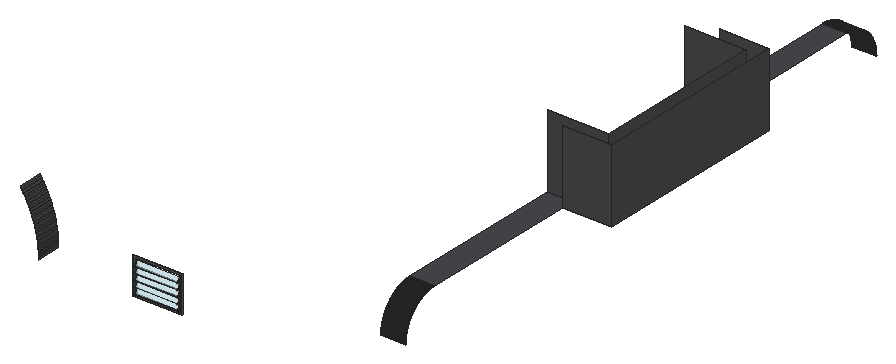
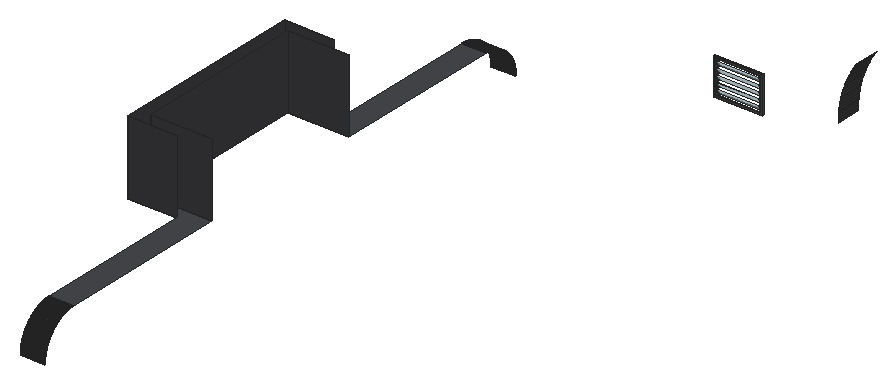
# SketchUp Ruby script. Lengths in inches.
U = 1.inch
M = Sketchup.active_model
def pt(a) = Geom::Point3d.new(a.map { |v| v * U })
def face(e, loops, mat)
  f = e.add_face(loops[0].map { |a| pt(a) })
  loops[1..].each { |l| e.add_face(l.map { |a| pt(a) }).erase! }
  f.material = f.back_material = mat if mat
  f
end
# faces: each face lists its corners as indices into pts; further lists are holes
def faces(e, pts, list, mat = nil) = list.each { |f| face(e, (f[0].is_a?(Array) ? f : [f]).map { |l| l.map { |i| pts[i] } }, mat) }
# xy, xz, yz: faces in a plane at the given z, y or x. An outline is a flat list of corners, or four numbers for a rectangle; further outlines are holes
def ring(l) = l.size == 4 ? [[l[0], l[1]], [l[2], l[1]], [l[2], l[3]], [l[0], l[3]]] : l.each_slice(2).to_a
def flat(e, list, mat, &to3) = list.each { |f| face(e, (f[0].is_a?(Array) ? f : [f]).map { |l| ring(l).map { |u, v| to3.(u, v) } }, mat) }
def xy(e, z, list, mat = nil) = flat(e, list, mat) { |x, y| [x, y, z] }
def xz(e, y, list, mat = nil) = flat(e, list, mat) { |x, z| [x, y, z] }
def yz(e, x, list, mat = nil) = flat(e, list, mat) { |y, z| [x, y, z] }
def lines(e, pts, list) = list.each { |a, b| e.add_line(pt(pts[a]), pt(pts[b])) }
# prism: a flat outline (further loops are holes) pulled along v
def prism(e, loops, v, mat = nil)
  f = face(e, loops, mat); d = Geom::Vector3d.new(v.map { |x| x * U })
  f.pushpull(f.normal.samedirection?(d) ? d.length : -d.length)
end
def box(e, o, s, mat = nil) = prism(e, [[o, [o[0] + s[0], o[1], o[2]], [o[0] + s[0], o[1] + s[1], o[2]], [o[0], o[1] + s[1], o[2]]]], [0, 0, s[2]], mat)
def at(x, y, z, deg = 0) = Geom::Transformation.translation(pt([x, y, z])) * Geom::Transformation.rotation(ORIGIN, Z_AXIS, deg.degrees)
def axes(o, x, y, z) = Geom::Transformation.new([*x, 0, *y, 0, *z, 0, *pt(o).to_a, 1])
def part(name) = M.definitions.add(name)
# library, detail: a bought-in or finely detailed component or shape, given as its bounding box
def library(name, o, s) = part(name).tap { |d| box(d.entities, o, s) }
def detail(e, o, s) = box(e.add_group.entities, o, s)
def put(e, d, t, mat = nil) = e.add_instance(d, t).tap { |i| i.material = mat if mat }
def group(e, t, mat = nil) = e.add_group.tap { |g| g.transformation = t; g.material = mat if mat }.entities
root = M.entities
M.materials.add("1432 AP 8245 TAR ROAD").color = [71, 72, 75]
M.materials.add("[Color M05]").color = [114, 114, 114]
M.materials.add("[Color M06]").color = [86, 86, 86]
M.materials.add("[Color M09]").color = [0, 0, 0]
M.materials.add("[Translucent Glass Safety]").color = [204, 235, 244]
M.materials["[Translucent Glass Safety]"].alpha = 0.5
M.materials.add("[Translucent Resin Crush Gray]").color = [209, 209, 209]
M.materials["[Translucent Resin Crush Gray]"].alpha = 0.8
c1 = part("Louvre blade clip")
prism(c1.entities,[[[0,0.85,29.12],[0,5.29,29.12],[0,5.29,0],[0,0,0],[0,0,9.17],[0,0.85,9.17],[0,0.85,0.85],[0,4.45,0.85],[0,4.45,28.27],[0,0.85,28.27]]],[0.5625,0,0],"[Color M09]")
c2 = part("Glass louvre blade")
p = [[0.14,0.43,0.55],[0.14,2.01,6.46],[0,2.375,6.37],[0,0.79,0.45],[29.62,0.79,0.45],[29.77,0.43,0.55],
  [29.77,2.01,6.46],[29.62,2.375,6.37]]
faces(c2.entities,p,[[0,1,2,3],[1,0,5,6],[4,7,6,5],[3,2,7,4],[2,1,6,7]],"[Translucent Glass Safety]")
faces(c2.entities,p,[[3,4,5,0]],"[Translucent Resin Crush Gray]")
put(c2.entities,c1,axes([29.2,0,0.28],[1,0,0],[0,0.19968,-0.0535],[0,0.06043,0.22552]))
put(c2.entities,c1,axes([-0.09,0.05,0.6],[1,0,0],[0,0.19968,-0.0535],[0,0.06043,0.22552]))
c3 = part("Window frame")
prism(c3.entities,[[[28.75,1.1875,0],[0,1.1875,0],[0,1.1875,36],[28.75,1.1875,36]],[[27.3,1.1875,1.45],[27.3,1.1875,34.55],[1.45,1.1875,34.55],[1.45,1.1875,1.45]]],[0,-1.1875,0],"[Color M06]")
c4 = part("Louvred window")
put(c4.entities,c2,axes([1.64,0,14.6],[0.837,0,0],[0,1,0],[0,0,0.7998]))
put(c4.entities,c2,axes([1.64,0,8.29],[0.837,0,0],[0,1,0],[0,0,0.7998]))
put(c4.entities,c2,axes([1.64,0,20.72],[0.837,0,0],[0,1,0],[0,0,0.7998]))
put(c4.entities,c2,axes([1.64,0,26.97],[0.837,0,0],[0,1,0],[0,0,0.7998]))
put(c4.entities,c2,axes([1.64,0,2.47],[0.837,0,0],[0,1,0],[0,0,0.7998]))
put(c4.entities,c3,axes([0,1.37,0],[0.98,0,0],[0,1,0],[0,0,1]),"[Color M05]")
c5 = part("BathRoom Window")
put(c5.entities,c4,at(2.44,2.32,-1.4375))
xy(root,419.79,[[573,160.9,585,161.13],[573,161.13,585,161.37],[573,161.37,573,245.37,603,245.37,603,329.37,573,329.37,573,413.37,585,413.37,585,335.37,609,335.37,609,239.37,585,239.37,585,161.37],[573,413.37,585,413.61],[573,413.61,585,413.84]],"1432 AP 8245 TAR ROAD")
xz(root,143.37,[[573,401.79,585,402.03]],"1432 AP 8245 TAR ROAD")
xz(root,239.37,[[585,419.79,609,455.79]],"1432 AP 8245 TAR ROAD")
xz(root,245.37,[[573,419.79,603,455.79]],"1432 AP 8245 TAR ROAD")
xz(root,329.37,[[573,419.79,603,455.79]],"1432 AP 8245 TAR ROAD")
xz(root,335.37,[[585,419.79,609,455.79]],"1432 AP 8245 TAR ROAD")
xz(root,431.36,[[573,402.26,585,402.5]],"1432 AP 8245 TAR ROAD")
xz(root,431.37,[[573,401.79,585,402.03]],"1432 AP 8245 TAR ROAD")
yz(root,444,[[95.37,410.79,107.37,411.46]],"1432 AP 8245 TAR ROAD")
yz(root,603,[[245.37,419.79,329.37,455.79]],"1432 AP 8245 TAR ROAD")
yz(root,609,[[239.37,419.79,335.37,455.79]],"1432 AP 8245 TAR ROAD")
p = [[573,143.37,402.03],[573,143.375,402.26],[585,143.375,402.26],[585,143.37,402.03],[573,431.36,402.26],[573,431.37,402.03],
  [585,431.37,402.03],[585,431.36,402.26],[573,143.38,402.5],[585,143.38,402.5],[573,143.39,402.73],[585,143.39,402.73],
  [573,431.35,402.73],[573,431.36,402.5],[585,431.36,402.5],[585,431.35,402.73],[573,143.41,402.97],[585,143.41,402.97],
  [573,431.33,402.97],[585,431.33,402.97],[573,143.43,403.2],[585,143.43,403.2],[573,431.3125,403.2],[585,431.3125,403.2],
  [573,143.45,403.4375],[585,143.45,403.4375],[573,431.29,403.4375],[585,431.29,403.4375],[573,143.47,403.67],[585,143.47,403.67],
  [573,431.27,403.67],[585,431.27,403.67],[573,143.49,403.91],[585,143.49,403.91],[573,431.25,403.91],[585,431.25,403.91],
  [573,143.52,404.14],[585,143.52,404.14],[573,431.22,404.14],[585,431.22,404.14],[573,143.56,404.375],[585,143.56,404.375],
  [573,431.18,404.375],[585,431.18,404.375],[573,143.59,404.61],[585,143.59,404.61],[573,431.15,404.61],[585,431.15,404.61],
  [573,143.63,404.84],[585,143.63,404.84],[573,431.11,404.84],[585,431.11,404.84],[573,143.67,405.07],[585,143.67,405.07],
  [573,431.07,405.07],[585,431.07,405.07],[573,143.72,405.3],[585,143.72,405.3],[573,431.02,405.3],[585,431.02,405.3],
  [573,143.76,405.53],[585,143.76,405.53],[573,430.98,405.53],[585,430.98,405.53],[573,143.8125,405.76],[585,143.8125,405.76],
  [573,430.93,405.76],[585,430.93,405.76],[573,143.87,405.99],[585,143.87,405.99],[573,430.87,405.99],[585,430.87,405.99],
  [573,143.92,406.22],[585,143.92,406.22],[573,430.82,406.22],[585,430.82,406.22],[573,143.98,406.45],[585,143.98,406.45],
  [573,430.76,406.45],[585,430.76,406.45],[573,144.05,406.68],[585,144.05,406.68],[573,430.69,406.68],[585,430.69,406.68],
  [573,144.11,406.9],[585,144.11,406.9],[573,430.63,406.9],[585,430.63,406.9],[573,144.18,407.13],[585,144.18,407.13],
  [573,430.56,407.13],[585,430.56,407.13],[573,144.25,407.35],[585,144.25,407.35],[573,430.49,407.35],[585,430.49,407.35],
  [573,144.33,407.58],[585,144.33,407.58],[573,430.41,407.58],[585,430.41,407.58],[573,144.4,407.8],[585,144.4,407.8],
  [573,430.34,407.8],[585,430.34,407.8],[573,144.48,408.02],[585,144.48,408.02],[573,430.26,408.02],[585,430.26,408.02],
  [573,144.57,408.24],[585,144.57,408.24],[573,430.17,408.24],[585,430.17,408.24],[573,144.65,408.46],[585,144.65,408.46],
  [573,430.09,408.46],[585,430.09,408.46],[573,144.74,408.68],[585,144.74,408.68],[573,430,408.68],[585,430,408.68],
  [573,144.83,408.9],[585,144.83,408.9],[573,429.91,408.9],[585,429.91,408.9],[573,144.93,409.11],[585,144.93,409.11],
  [573,429.8125,409.11],[585,429.8125,409.11],[573,145.02,409.33],[585,145.02,409.33],[573,429.72,409.33],[585,429.72,409.33],
  [573,145.125,409.54],[585,145.125,409.54],[573,429.62,409.54],[585,429.62,409.54],[573,145.23,409.75],[585,145.23,409.75],
  [573,429.51,409.75],[585,429.51,409.75],[573,145.33,409.96],[585,145.33,409.96],[573,429.41,409.96],[585,429.41,409.96],
  [573,145.44,410.17],[585,145.44,410.17],[573,429.3,410.17],[585,429.3,410.17],[573,145.55,410.38],[585,145.55,410.38],
  [573,429.1875,410.38],[585,429.1875,410.38],[573,145.67,410.59],[585,145.67,410.59],[573,429.07,410.59],[585,429.07,410.59],
  [573,145.78,410.79],[585,145.78,410.79],[573,428.96,410.79],[585,428.96,410.79],[573,145.9,411],[585,145.9,411],
  [573,428.84,411],[585,428.84,411],[573,146.02,411.2],[585,146.02,411.2],[573,428.72,411.2],[585,428.72,411.2],
  [573,146.15,411.4],[585,146.15,411.4],[573,428.59,411.4],[585,428.59,411.4],[573,146.27,411.6],[585,146.27,411.6],
  [573,428.47,411.6],[585,428.47,411.6],[444,107.37,411.46],[443.98,107.37,412.13],[443.98,95.37,412.13],[444,95.37,411.46],
  [573,146.4,411.79],[585,146.4,411.79],[573,428.34,411.79],[585,428.34,411.79],[573,146.54,411.99],[585,146.54,411.99],
  [573,428.2,411.99],[585,428.2,411.99],[573,146.67,412.18],[585,146.67,412.18],[573,428.07,412.18],[585,428.07,412.18],
  [443.96,107.37,412.79],[443.96,95.37,412.79],[573,146.81,412.37],[585,146.81,412.37],[573,427.93,412.37],[585,427.93,412.37],
  [573,146.95,412.5625],[585,146.95,412.5625],[573,427.79,412.5625],[585,427.79,412.5625],[573,147.09,412.75],[585,147.09,412.75],
  [573,427.65,412.75],[585,427.65,412.75],[573,147.23,412.9375],[585,147.23,412.9375],[573,427.51,412.9375],[585,427.51,412.9375],
  [443.93,107.37,413.46],[443.93,95.37,413.46],[573,147.38,413.12],[585,147.38,413.12],[573,427.36,413.12],[585,427.36,413.12],
  [573,147.53,413.3],[585,147.53,413.3],[573,427.21,413.3],[585,427.21,413.3],[573,147.68,413.48],[585,147.68,413.48],
  [573,427.06,413.48],[585,427.06,413.48],[443.89,107.37,414.13],[443.89,95.37,414.13],[573,147.84,413.66],[585,147.84,413.66],
  [573,426.9,413.66],[585,426.9,413.66],[573,147.99,413.84],[585,147.99,413.84],[573,426.75,413.84],[585,426.75,413.84],
  [573,148.15,414.01],[585,148.15,414.01],[573,426.59,414.01],[585,426.59,414.01],[573,148.3125,414.18],[585,148.3125,414.18],
  [573,426.43,414.18],[585,426.43,414.18],[443.84,107.37,414.79],[443.84,95.37,414.79],[573,148.48,414.35],[585,148.48,414.35],
  [573,426.26,414.35],[585,426.26,414.35],[573,148.64,414.52],[585,148.64,414.52],[573,426.1,414.52],[585,426.1,414.52],
  [573,148.81,414.69],[585,148.81,414.69],[573,425.93,414.69],[585,425.93,414.69],[573,148.98,414.85],[585,148.98,414.85],
  [573,425.76,414.85],[585,425.76,414.85],[443.79,107.37,415.46],[443.79,95.37,415.46],[573,149.15,415.01],[585,149.15,415.01],
  [573,425.59,415.01],[585,425.59,415.01],[573,149.33,415.17],[585,149.33,415.17],[573,425.41,415.17],[585,425.41,415.17],
  [573,149.5,415.33],[585,149.5,415.33],[573,425.24,415.33],[585,425.24,415.33],[573,149.68,415.48],[585,149.68,415.48],
  [573,425.06,415.48],[585,425.06,415.48],[443.72,107.37,416.125],[443.72,95.37,416.125],[573,149.86,415.63],[585,149.86,415.63],
  [573,424.88,415.63],[585,424.88,415.63],[573,150.04,415.78],[585,150.04,415.78],[573,424.7,415.78],[585,424.7,415.78],
  [573,150.23,415.93],[585,150.23,415.93],[573,424.51,415.93],[585,424.51,415.93],[573,150.41,416.07],[585,150.41,416.07],
  [573,424.33,416.07],[585,424.33,416.07],[443.65,107.37,416.79],[443.65,95.37,416.79],[573,150.6,416.21],[585,150.6,416.21],
  [573,424.14,416.21],[585,424.14,416.21],[573,150.79,416.35],[585,150.79,416.35],[573,423.95,416.35],[585,423.95,416.35],
  [573,150.98,416.49],[585,150.98,416.49],[573,423.76,416.49],[585,423.76,416.49],[573,151.17,416.625],[585,151.17,416.625],
  [573,423.57,416.625],[585,423.57,416.625],[573,151.37,416.76],[585,151.37,416.76],[573,423.37,416.76],[585,423.37,416.76],
  [443.5625,107.37,417.45],[443.5625,95.37,417.45],[573,151.57,416.89],[585,151.57,416.89],[573,423.17,416.89],[585,423.17,416.89],
  [573,151.76,417.02],[585,151.76,417.02],[573,422.97,417.02],[585,422.97,417.02],[573,151.96,417.14],[585,151.96,417.14],
  [573,422.77,417.14],[585,422.77,417.14],[573,152.17,417.26],[585,152.17,417.26],[573,422.57,417.26],[585,422.57,417.26],
  [573,152.37,417.38],[585,152.37,417.38],[573,422.37,417.38],[585,422.37,417.38],[443.47,107.37,418.11],[443.47,95.37,418.11],
  [573,152.57,417.5],[585,152.57,417.5],[573,422.17,417.5],[585,422.17,417.5],[573,152.78,417.61],[585,152.78,417.61],
  [573,421.96,417.61],[585,421.96,417.61],[573,152.99,417.72],[585,152.99,417.72],[573,421.75,417.72],[585,421.75,417.72],
  [573,153.2,417.83],[585,153.2,417.83],[573,421.54,417.83],[585,421.54,417.83],[573,153.41,417.9375],[585,153.41,417.9375],
  [573,421.33,417.9375],[585,421.33,417.9375],[573,153.62,418.04],[585,153.62,418.04],[573,421.12,418.04],[585,421.12,418.04],
  [573,153.83,418.14],[585,153.83,418.14],[573,420.91,418.14],[585,420.91,418.14],[443.37,107.37,418.77],[443.37,95.37,418.77],
  [573,154.05,418.24],[585,154.05,418.24],[573,420.69,418.24],[585,420.69,418.24],[573,154.26,418.33],[585,154.26,418.33],
  [573,420.48,418.33],[585,420.48,418.33],[573,154.48,418.42],[585,154.48,418.42],[573,420.26,418.42],[585,420.26,418.42],
  [573,154.7,418.51],[585,154.7,418.51],[573,420.04,418.51],[585,420.04,418.51],[573,154.92,418.6],[585,154.92,418.6],
  [573,419.82,418.6],[585,419.82,418.6],[573,155.14,418.68],[585,155.14,418.68],[573,419.6,418.68],[585,419.6,418.68],
  [573,155.36,418.76],[585,155.36,418.76],[573,419.38,418.76],[585,419.38,418.76],[443.26,107.37,419.43],[443.26,95.37,419.43],
  [573,155.58,418.84],[585,155.58,418.84],[573,155.81,418.91],[585,155.81,418.91],[573,418.93,418.91],[573,419.16,418.84],
  [585,419.16,418.84],[585,418.93,418.91],[573,156.03,418.98],[585,156.03,418.98],[573,418.71,418.98],[585,418.71,418.98],
  [573,156.26,419.05],[585,156.26,419.05],[573,418.48,419.05],[585,418.48,419.05],[573,156.48,419.12],[585,156.48,419.12],
  [573,156.71,419.18],[585,156.71,419.18],[573,418.03,419.18],[573,418.26,419.12],[585,418.26,419.12],[585,418.03,419.18],
  [573,156.9375,419.24],[585,156.9375,419.24],[573,157.17,419.29],[585,157.17,419.29],[573,417.57,419.29],[573,417.8,419.24],
  [585,417.8,419.24],[585,417.57,419.29],[573,157.4,419.35],[585,157.4,419.35],[573,157.63,419.4],[585,157.63,419.4],
  [573,417.11,419.4],[573,417.34,419.35],[585,417.34,419.35],[585,417.11,419.4],[443.15,107.37,420.09],[443.15,95.37,420.09],
  [573,157.86,419.45],[585,157.86,419.45],[573,158.09,419.49],[585,158.09,419.49],[573,416.65,419.49],[573,416.88,419.45],
  [585,416.88,419.45],[585,416.65,419.49],[573,158.32,419.53],[585,158.32,419.53],[573,158.55,419.57],[585,158.55,419.57],
  [573,416.1875,419.57],[573,416.42,419.53],[585,416.42,419.53],[585,416.1875,419.57],[573,158.79,419.61],[585,158.79,419.61],
  [573,159.02,419.64],[585,159.02,419.64],[573,159.25,419.67],[585,159.25,419.67],[573,415.49,419.67],[573,415.72,419.64],
  [585,415.72,419.64],[585,415.49,419.67],[573,415.95,419.61],[585,415.95,419.61],[573,159.49,419.69],[585,159.49,419.69],
  [573,159.72,419.72],[585,159.72,419.72],[573,159.96,419.74],[585,159.96,419.74],[573,160.19,419.75],[585,160.19,419.75],
  [573,414.55,419.75],[573,414.78,419.74],[585,414.78,419.74],[585,414.55,419.75],[573,415.02,419.72],[585,415.02,419.72],
  [573,415.25,419.69],[585,415.25,419.69],[573,160.43,419.77],[585,160.43,419.77],[573,160.66,419.78],[585,160.66,419.78],
  [573,160.9,419.79],[585,160.9,419.79],[573,413.84,419.79],[573,414.08,419.78],[585,414.08,419.78],[585,413.84,419.79],
  [573,414.3125,419.77],[585,414.3125,419.77],[443.02,107.37,420.74],[443.02,95.37,420.74],[442.89,107.37,421.4],[442.89,95.37,421.4],
  [442.74,107.37,422.05],[442.74,95.37,422.05],[442.59,107.37,422.7],[442.59,95.37,422.7],[442.43,107.37,423.35],[442.43,95.37,423.35],
  [442.26,107.37,423.99],[442.26,95.37,423.99],[442.09,107.37,424.64],[442.09,95.37,424.64],[441.9,107.37,425.28],[441.9,95.37,425.28],
  [441.71,107.37,425.92],[441.71,95.37,425.92],[441.5,107.37,426.55],[441.5,95.37,426.55],[441.29,107.37,427.19],[441.29,95.37,427.19],
  [441.07,107.37,427.82],[441.07,95.37,427.82],[440.85,107.37,428.44],[440.85,95.37,428.44],[440.61,107.37,429.07],[440.61,95.37,429.07],
  [440.37,107.37,429.69],[440.37,95.37,429.69],[440.12,107.37,430.31],[440.12,95.37,430.31],[439.86,107.37,430.92],[439.86,95.37,430.92],
  [439.59,107.37,431.54],[439.59,95.37,431.54],[439.32,107.37,432.14],[439.32,95.37,432.14],[439.03,107.37,432.75],[439.03,95.37,432.75],
  [438.74,107.37,433.35],[438.74,95.37,433.35],[438.44,107.37,433.95],[438.44,95.37,433.95],[438.13,107.37,434.54],[438.13,95.37,434.54],
  [437.82,107.37,435.13],[437.82,95.37,435.13],[437.5,107.37,435.71],[437.5,95.37,435.71],[437.17,107.37,436.29],[437.17,95.37,436.29],
  [436.83,107.37,436.87],[436.83,95.37,436.87],[436.48,107.37,437.4375],[436.48,95.37,437.4375],[436.13,107.37,438.01],[436.13,95.37,438.01],
  [435.77,107.37,438.57],[435.77,95.37,438.57],[435.4,107.37,439.125],[435.4,95.37,439.125],[435.03,107.37,439.68],[435.03,95.37,439.68]]
faces(root,p,[[0,1,2,3],[4,5,6,7],[1,8,9,2],[8,10,11,9],[12,13,14,15],[10,16,17,11],[18,12,15,19],[16,20,21,17],
  [22,18,19,23],[20,24,25,21],[26,22,23,27],[24,28,29,25],[30,26,27,31],[28,32,33,29],[34,30,31,35],[32,36,37,33],
  [38,34,35,39],[36,40,41,37],[42,38,39,43],[40,44,45,41],[46,42,43,47],[44,48,49,45],[50,46,47,51],[48,52,53,49],
  [54,50,51,55],[52,56,57,53],[58,54,55,59],[56,60,61,57],[62,58,59,63],[60,64,65,61],[66,62,63,67],[64,68,69,65],
  [70,66,67,71],[68,72,73,69],[74,70,71,75],[72,76,77,73],[78,74,75,79],[76,80,81,77],[82,78,79,83],[80,84,85,81],
  [86,82,83,87],[84,88,89,85],[90,86,87,91],[88,92,93,89],[94,90,91,95],[92,96,97,93],[98,94,95,99],[96,100,101,97],
  [102,98,99,103],[100,104,105,101],[106,102,103,107],[104,108,109,105],[110,106,107,111],[108,112,113,109],[114,110,111,115],[112,116,117,113],
  [118,114,115,119],[116,120,121,117],[122,118,119,123],[120,124,125,121],[126,122,123,127],[124,128,129,125],[130,126,127,131],[128,132,133,129],
  [134,130,131,135],[132,136,137,133],[138,134,135,139],[136,140,141,137],[142,138,139,143],[140,144,145,141],[146,142,143,147],[144,148,149,145],
  [150,146,147,151],[148,152,153,149],[154,150,151,155],[152,156,157,153],[158,154,155,159],[156,160,161,157],[162,158,159,163],[160,164,165,161],
  [166,162,163,167],[164,168,169,165],[170,166,167,171],[168,172,173,169],[174,170,171,175],[176,177,178,179],[172,180,181,173],[182,174,175,183],
  [180,184,185,181],[186,182,183,187],[184,188,189,185],[190,186,187,191],[177,192,193,178],[188,194,195,189],[196,190,191,197],[194,198,199,195],
  [200,196,197,201],[198,202,203,199],[204,200,201,205],[202,206,207,203],[208,204,205,209],[192,210,211,193],[206,212,213,207],[214,208,209,215],
  [212,216,217,213],[218,214,215,219],[216,220,221,217],[222,218,219,223],[210,224,225,211],[220,226,227,221],[228,222,223,229],[226,230,231,227],
  [232,228,229,233],[230,234,235,231],[236,232,233,237],[234,238,239,235],[240,236,237,241],[224,242,243,225],[238,244,245,239],[246,240,241,247],
  [244,248,249,245],[250,246,247,251],[248,252,253,249],[254,250,251,255],[252,256,257,253],[258,254,255,259],[242,260,261,243],[256,262,263,257],
  [264,258,259,265],[262,266,267,263],[268,264,265,269],[266,270,271,267],[272,268,269,273],[270,274,275,271],[276,272,273,277],[260,278,279,261],
  [274,280,281,275],[282,276,277,283],[280,284,285,281],[286,282,283,287],[284,288,289,285],[290,286,287,291],[288,292,293,289],[294,290,291,295],
  [278,296,297,279],[292,298,299,293],[300,294,295,301],[298,302,303,299],[304,300,301,305],[302,306,307,303],[308,304,305,309],[306,310,311,307],
  [312,308,309,313],[310,314,315,311],[316,312,313,317],[296,318,319,297],[314,320,321,315],[322,316,317,323],[320,324,325,321],[326,322,323,327],
  [324,328,329,325],[330,326,327,331],[328,332,333,329],[334,330,331,335],[332,336,337,333],[338,334,335,339],[318,340,341,319],[336,342,343,337],
  [344,338,339,345],[342,346,347,343],[348,344,345,349],[346,350,351,347],[352,348,349,353],[350,354,355,351],[356,352,353,357],[354,358,359,355],
  [360,356,357,361],[358,362,363,359],[364,360,361,365],[362,366,367,363],[368,364,365,369],[340,370,371,341],[366,372,373,367],[374,368,369,375],
  [372,376,377,373],[378,374,375,379],[376,380,381,377],[382,378,379,383],[380,384,385,381],[386,382,383,387],[384,388,389,385],[390,386,387,391],
  [388,392,393,389],[394,390,391,395],[392,396,397,393],[398,394,395,399],[370,400,401,371],[396,402,403,397],[402,404,405,403],[406,407,408,409],
  [407,398,399,408],[404,410,411,405],[412,406,409,413],[410,414,415,411],[416,412,413,417],[414,418,419,415],[418,420,421,419],[422,423,424,425],
  [423,416,417,424],[420,426,427,421],[426,428,429,427],[430,431,432,433],[431,422,425,432],[428,434,435,429],[434,436,437,435],[438,439,440,441],
  [439,430,433,440],[400,442,443,401],[436,444,445,437],[444,446,447,445],[448,449,450,451],[449,438,441,450],[446,452,453,447],[452,454,455,453],
  [456,457,458,459],[457,448,451,458],[454,460,461,455],[460,462,463,461],[462,464,465,463],[466,467,468,469],[467,470,471,468],[470,456,459,471],
  [464,472,473,465],[472,474,475,473],[474,476,477,475],[476,478,479,477],[480,481,482,483],[481,484,485,482],[484,486,487,485],[486,466,469,487],
  [478,488,489,479],[488,490,491,489],[490,492,493,491],[494,495,496,497],[495,498,499,496],[498,480,483,499],[442,500,501,443],[500,502,503,501],
  [502,504,505,503],[504,506,507,505],[506,508,509,507],[508,510,511,509],[510,512,513,511],[512,514,515,513],[514,516,517,515],[516,518,519,517],
  [518,520,521,519],[520,522,523,521],[522,524,525,523],[524,526,527,525],[526,528,529,527],[528,530,531,529],[530,532,533,531],[532,534,535,533],
  [534,536,537,535],[536,538,539,537],[538,540,541,539],[540,542,543,541],[542,544,545,543],[544,546,547,545],[546,548,549,547],[548,550,551,549],
  [550,552,553,551],[552,554,555,553],[554,556,557,555],[556,558,559,557],[558,560,561,559],[560,562,563,561]],"1432 AP 8245 TAR ROAD")
put(root,c5,axes([477.92,106.21,402.51],[0.85182,0,0],[0,0.5,0],[0,0,0.5]))
